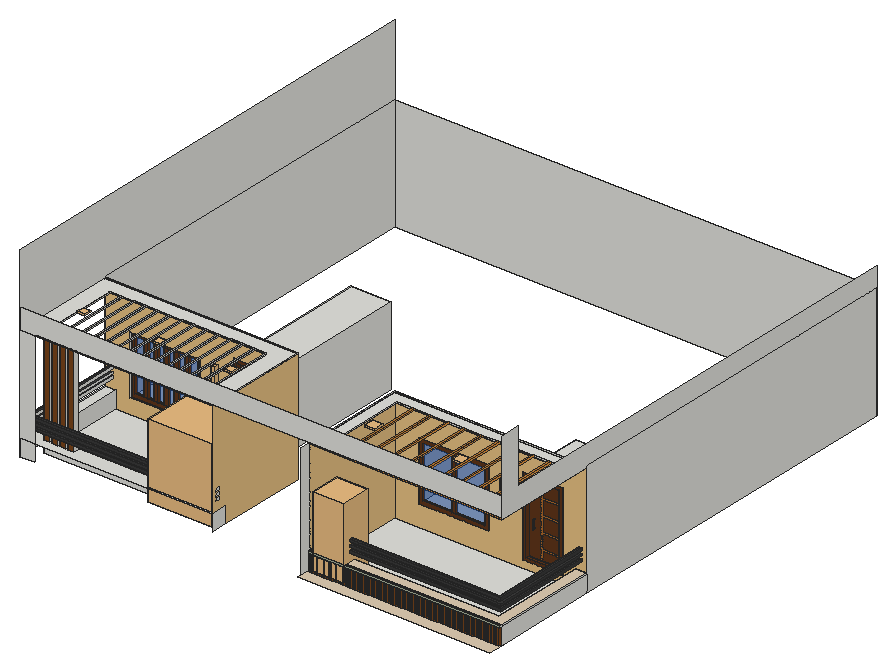
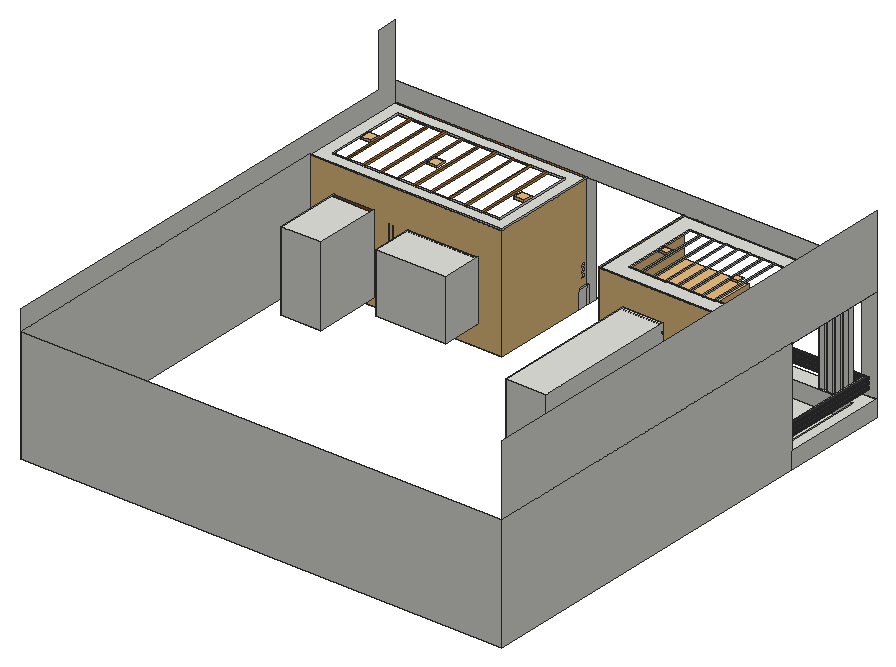
# SketchUp Ruby script. Lengths in inches.
U = 1.inch
M = Sketchup.active_model
def pt(a) = Geom::Point3d.new(a.map { |v| v * U })
def face(e, loops, mat)
  f = e.add_face(loops[0].map { |a| pt(a) })
  loops[1..].each { |l| e.add_face(l.map { |a| pt(a) }).erase! }
  f.material = f.back_material = mat if mat
  f
end
# faces: each face lists its corners as indices into pts; further lists are holes
def faces(e, pts, list, mat = nil) = list.each { |f| face(e, (f[0].is_a?(Array) ? f : [f]).map { |l| l.map { |i| pts[i] } }, mat) }
# xy, xz, yz: faces in a plane at the given z, y or x. An outline is a flat list of corners, or four numbers for a rectangle; further outlines are holes
def ring(l) = l.size == 4 ? [[l[0], l[1]], [l[2], l[1]], [l[2], l[3]], [l[0], l[3]]] : l.each_slice(2).to_a
def flat(e, list, mat, &to3) = list.each { |f| face(e, (f[0].is_a?(Array) ? f : [f]).map { |l| ring(l).map { |u, v| to3.(u, v) } }, mat) }
def xy(e, z, list, mat = nil) = flat(e, list, mat) { |x, y| [x, y, z] }
def xz(e, y, list, mat = nil) = flat(e, list, mat) { |x, z| [x, y, z] }
def yz(e, x, list, mat = nil) = flat(e, list, mat) { |y, z| [x, y, z] }
def lines(e, pts, list) = list.each { |a, b| e.add_line(pt(pts[a]), pt(pts[b])) }
# prism: a flat outline (further loops are holes) pulled along v
def prism(e, loops, v, mat = nil)
  f = face(e, loops, mat); d = Geom::Vector3d.new(v.map { |x| x * U })
  f.pushpull(f.normal.samedirection?(d) ? d.length : -d.length)
end
def box(e, o, s, mat = nil) = prism(e, [[o, [o[0] + s[0], o[1], o[2]], [o[0] + s[0], o[1] + s[1], o[2]], [o[0], o[1] + s[1], o[2]]]], [0, 0, s[2]], mat)
def at(x, y, z, deg = 0) = Geom::Transformation.translation(pt([x, y, z])) * Geom::Transformation.rotation(ORIGIN, Z_AXIS, deg.degrees)
def axes(o, x, y, z) = Geom::Transformation.new([*x, 0, *y, 0, *z, 0, *pt(o).to_a, 1])
def part(name) = M.definitions.add(name)
# library, detail: a bought-in or finely detailed component or shape, given as its bounding box
def library(name, o, s) = part(name).tap { |d| box(d.entities, o, s) }
def detail(e, o, s) = box(e.add_group.entities, o, s)
def put(e, d, t, mat = nil) = e.add_instance(d, t).tap { |i| i.material = mat if mat }
def group(e, t, mat = nil) = e.add_group.tap { |g| g.transformation = t; g.material = mat if mat }.entities
root = M.entities
M.materials.add("Generic\#1").color = [121, 68, 27]
M.materials.add("Generic\#4").color = [232, 149, 60]
M.materials.add("Generic\#5").color = [233, 194, 132]
M.materials.add("Generic\#6").color = [223, 205, 179]
M.materials.add("Generic\#8").color = [168, 180, 155]
M.materials.add("[Color M05]").color = [114, 114, 114]
M.materials.add("[Color M07]").color = [58, 58, 58]
M.materials.add("[Translucent Glass Blue]").color = [28, 83, 181]
M.materials["[Translucent Glass Blue]"].alpha = 0.5
M.materials.add("[Wood Bamboo]").color = [177, 105, 43]
M.materials.add("[Wood Cherry Original]").color = [96, 54, 26]
c1 = part("Group\#10")
xy(c1.entities,17.5625,[[0,0,2,2]])
xz(c1.entities,0,[[0,0,2,17.5625]])
yz(c1.entities,2,[[0,0,2,17.5625]])
c2 = library("Group_2",[-1.28,-0.39,0],[21.22,20.51,48.44])
c3 = library("Flora+17",[-57.52,158.6,-38.64],[66.99,62.88,77.28])
c4 = part("Group\#5")
xy(c4.entities,0,[[0,0,41.8125,3.4375]],"[Wood Cherry Original]")
xy(c4.entities,3.53,[[3.53,0,38.28,3.4375]],"[Wood Cherry Original]")
xy(c4.entities,31.39,[[9.28,1.32,9.97,3.4375]])
xy(c4.entities,32.05,[[9.29,1.98,9.98,3.4375]],"[Color M05]")
xy(c4.entities,39.77,[[9.29,1.98,9.98,3.4375]])
xy(c4.entities,40.43,[[9.28,1.32,9.97,3.4375]],"[Color M05]")
xy(c4.entities,79.47,[[3.53,0,38.28,3.4375]],"[Wood Cherry Original]")
xy(c4.entities,83,[[0,0,41.8125,3.4375]],"[Wood Cherry Original]")
xz(c4.entities,0,[[[0,0,41.8125,83],[3.53,3.53,38.28,79.47]]],"[Wood Cherry Original]")
xz(c4.entities,1.32,[[9.28,31.39,9.97,40.43]],"[Color M05]")
xz(c4.entities,1.98,[[9.29,32.05,9.98,39.77]],"[Color M05]")
xz(c4.entities,3.4375,[[9.29,39.77,9.28,40.43,9.97,40.43,9.98,39.77]])
xz(c4.entities,3.4375,[[16.22,3.53,17.74,3.53,17.74,13.29,38.28,13.29,38.28,15.09,17.74,15.09,17.74,29.41,38.28,29.41,38.28,31.22,17.74,31.22,17.74,45.54,38.28,45.54,38.28,47.34,17.74,47.34,17.74,61.66,38.28,61.66,38.28,63.47,17.74,63.47,17.74,79.47,16.22,79.47]],"[Wood Bamboo]")
xz(c4.entities,3.4375,[[[0,0,41.8125,83],[3.53,3.53,38.28,79.47]],[[3.53,3.53,16.22,79.47],[9.29,39.77,9.28,40.43,9.97,40.43,9.98,39.77],[9.28,31.39,9.29,32.05,9.98,32.05,9.97,31.39]],[17.74,3.53,38.28,13.29],[17.74,15.09,38.28,29.41],[17.74,31.22,38.28,45.54],
  [17.74,47.34,38.28,61.66],[17.74,63.47,38.28,79.47]],"[Wood Cherry Original]")
yz(c4.entities,0,[[0,0,3.4375,83]],"[Wood Cherry Original]")
yz(c4.entities,3.53,[[0,3.53,3.4375,79.47]],"[Wood Cherry Original]")
yz(c4.entities,38.28,[[0,3.53,3.4375,79.47]],"[Wood Cherry Original]")
yz(c4.entities,41.8125,[[0,0,3.4375,83]],"[Wood Cherry Original]")
p = [[9.28,1.32,40.43],[9.29,1.98,39.77],[9.29,1.98,32.05],[9.28,1.32,31.39],[9.29,3.4375,32.05],[9.28,3.4375,31.39],
  [9.98,1.98,39.77],[9.97,1.32,40.43],[9.97,1.32,31.39],[9.98,1.98,32.05],[9.97,3.4375,31.39],[9.98,3.4375,32.05],
  [9.28,3.4375,40.43],[9.29,3.4375,39.77],[9.98,3.4375,39.77],[9.97,3.4375,40.43],[9.625,3.4375,40.13],[9.625,1.625,40.13],
  [9.625,1.625,31.69],[9.625,3.4375,31.69]]
faces(c4.entities,p,[[0,1,2,3],[3,2,4,5],[6,7,8,9],[9,8,10,11],[12,13,1,0],[14,15,7,6]],"[Color M05]")
lines(c4.entities,p,[[16,17],[18,19],[17,18]])
c5 = part("Group\#3")
xy(c5.entities,0,[[0,0,81.86,2.5]],"[Wood Cherry Original]")
xy(c5.entities,4.12,[[4.12,0,13.68,2.5],[13.68,0,18.93,2.5],[18.93,0,25.68,2.5],[25.68,0,30.93,2.5],[30.93,0,37.68,2.5],
  [37.68,0,42.93,2.5],[42.93,0,49.68,2.5],[49.68,0,54.93,2.5],[54.93,0,61.68,2.5],[61.68,0,66.93,2.5],
  [66.93,0,77.74,2.5]],"[Wood Cherry Original]")
xy(c5.entities,66.49,[[4.12,0,13.68,2.5],[13.68,0,18.93,2.5],[18.93,0,25.68,2.5],[25.68,0,30.93,2.5],[30.93,0,37.68,2.5],
  [37.68,0,42.93,2.5],[42.93,0,49.68,2.5],[49.68,0,54.93,2.5],[54.93,0,61.68,2.5],[61.68,0,66.93,2.5],
  [66.93,0,77.74,2.5]],"[Wood Cherry Original]")
xy(c5.entities,70.61,[[0,0,81.86,2.5]],"[Wood Cherry Original]")
xz(c5.entities,0,[[[0,0,81.86,70.61],[4.12,4.12,77.74,66.49]],[13.68,4.12,18.93,66.49],[25.68,4.12,30.93,66.49],[37.68,4.12,42.93,66.49],[49.68,4.12,54.93,66.49],
  [61.68,4.12,66.93,66.49]],"[Wood Cherry Original]")
xz(c5.entities,2.5,[[4.12,4.12,13.68,66.49],[18.93,4.12,25.68,66.49],[30.93,4.12,37.68,66.49],[42.93,4.12,49.68,66.49],[54.93,4.12,61.68,66.49],
  [66.93,4.12,77.74,66.49]],"[Translucent Glass Blue]")
xz(c5.entities,2.5,[[[0,0,81.86,70.61],[4.12,4.12,77.74,66.49]]],"[Wood Cherry Original]")
yz(c5.entities,0,[[0,0,2.5,70.61]],"[Wood Cherry Original]")
yz(c5.entities,4.12,[[0,4.12,2.5,66.49]],"[Wood Cherry Original]")
yz(c5.entities,13.68,[[0,4.12,2.5,66.49]],"[Wood Cherry Original]")
yz(c5.entities,18.93,[[0,4.12,2.5,66.49]],"[Wood Cherry Original]")
yz(c5.entities,25.68,[[0,4.12,2.5,66.49]],"[Wood Cherry Original]")
yz(c5.entities,30.93,[[0,4.12,2.5,66.49]],"[Wood Cherry Original]")
yz(c5.entities,37.68,[[0,4.12,2.5,66.49]],"[Wood Cherry Original]")
yz(c5.entities,42.93,[[0,4.12,2.5,66.49]],"[Wood Cherry Original]")
yz(c5.entities,49.68,[[0,4.12,2.5,66.49]],"[Wood Cherry Original]")
yz(c5.entities,54.93,[[0,4.12,2.5,66.49]],"[Wood Cherry Original]")
yz(c5.entities,61.68,[[0,4.12,2.5,66.49]],"[Wood Cherry Original]")
yz(c5.entities,66.93,[[0,4.12,2.5,66.49]],"[Wood Cherry Original]")
yz(c5.entities,77.74,[[0,4.12,2.5,66.49]],"[Wood Cherry Original]")
yz(c5.entities,81.86,[[0,0,2.5,70.61]],"[Wood Cherry Original]")
c6 = part("Group\#4")
xy(c6.entities,0,[[0,0,73.625,2.0625]],"[Wood Cherry Original]")
xy(c6.entities,3.98,[[35.0625,0,38.75,2.0625]])
xy(c6.entities,3.98,[[3.98,0,35.0625,2.0625],[38.75,0,69.64,2.0625]],"[Wood Cherry Original]")
xy(c6.entities,58.39,[[35.0625,0,38.75,2.0625]])
xy(c6.entities,58.39,[[3.98,0,35.0625,2.0625],[38.75,0,69.64,2.0625]],"[Wood Cherry Original]")
xy(c6.entities,62.375,[[0,0,73.625,2.0625]],"[Wood Cherry Original]")
xz(c6.entities,0,[[[0,0,73.625,62.375],[3.98,3.98,69.64,58.39]],[35.0625,3.98,38.75,58.39]],"[Wood Cherry Original]")
xz(c6.entities,2.0625,[[[0,0,73.625,62.375],[3.98,3.98,69.64,58.39]]])
xz(c6.entities,2.0625,[[3.98,3.98,35.0625,58.39],[38.75,3.98,69.64,58.39]],"[Translucent Glass Blue]")
yz(c6.entities,0,[[0,0,2.0625,62.375]],"[Wood Cherry Original]")
yz(c6.entities,3.98,[[0,3.98,2.0625,58.39]],"[Wood Cherry Original]")
yz(c6.entities,35.0625,[[0,3.98,2.0625,58.39]],"[Wood Cherry Original]")
yz(c6.entities,38.75,[[0,3.98,2.0625,58.39]],"[Wood Cherry Original]")
yz(c6.entities,69.64,[[0,3.98,2.0625,58.39]],"[Wood Cherry Original]")
yz(c6.entities,73.625,[[0,0,2.0625,62.375]],"[Wood Cherry Original]")
c7 = library("Lamp Wall Outdoor 94-02",[-1.89,-4.65,-3.17],[3.78,4.65,6.35])
c8 = library("Tlon Light 450 Ceiling 152 006",[-8.86,-8.86,-3.78],[17.72,17.72,3.56])
xy(root,422.625,[[306.09,52.5625,308.09,54.5625],[306.09,54.5625,306.09,65.5625,496.1875,65.5625,496.1875,166.1875,507.875,166.1875,507.875,54.5625],[306.09,65.5625,496.1875,166.1875],[13.4375,71.3125,204.09,166.1875]])
xy(root,422.625,[[306.09,39.375,507.875,39.375,507.875,54.5625,308.09,54.5625,308.09,52.5625,306.09,52.5625]],"Generic\#6")
xy(root,430.43,[[440.99,166.1875,482.8,235.75]])
xy(root,430.93,[[137.36,166.1875,179.17,320.375]])
xy(root,438.15,[[27.78,166.1875,101.4,224.375]])
xy(root,440.1875,[[306.09,51.8125,308.09,54.5625],[308.09,51.8125,507.875,54.5625],[[2.3125,54.5625,204.09,54.5625,204.09,71.3125,13.4375,71.3125,13.4375,166.1875,2.3125,166.1875],[19.41,64.07,25.6,69.2],[27.85,64.07,34.03,69.2],[36.28,64.07,42.47,69.2],[44.72,64.07,50.91,69.2]],[306.09,54.5625,306.09,65.5625,496.1875,65.5625,496.1875,166.1875,507.875,166.1875,507.875,54.5625]])
xy(root,441.875,[[306.09,54.5625,507.875,54.5625,507.875,166.1875,496.1875,166.1875,496.1875,65.5625,306.09,65.5625]],"Generic\#6")
xy(root,441.875,[[306.09,51.8125,507.875,54.5625]],"Generic\#8")
xy(root,444.9,[[331.4,166.1875,405.03,208.8125]])
xy(root,449.75,[[6.99,59.18,6.99,166.1875,10.24,166.1875,10.24,62.43,204.09,62.43,204.09,59.18]],"[Color M07]")
xy(root,450.64,[[306.09,58.77,306.09,61.77,500.32,61.77,500.32,166.1875,503.32,166.1875,503.32,58.77]],"[Color M07]")
xy(root,452.5,[[6.99,59.18,204.09,59.18,204.09,62.43,10.24,62.43,10.24,166.1875,6.99,166.1875]],"[Color M07]")
xy(root,453.2,[[306.09,58.77,503.32,58.77,503.32,166.1875,500.32,166.1875,500.32,61.77,306.09,61.77]],"[Color M07]")
xy(root,454,[[6.99,59.18,6.99,166.1875,10.24,166.1875,10.24,62.43,204.09,62.43,204.09,59.18]],"[Color M07]")
xy(root,456.01,[[306.09,58.77,306.09,61.77,500.32,61.77,500.32,166.1875,503.32,166.1875,503.32,58.77]],"[Color M07]")
xy(root,456.75,[[6.99,59.18,204.09,59.18,204.09,62.43,10.24,62.43,10.24,166.1875,6.99,166.1875]],"[Color M07]")
xy(root,458.58,[[306.09,58.77,503.32,58.77,503.32,166.1875,500.32,166.1875,500.32,61.77,306.09,61.77]],"[Color M07]")
xy(root,458.75,[[6.99,59.18,6.99,166.1875,10.24,166.1875,10.24,62.43,204.09,62.43,204.09,59.18]],"[Color M07]")
xy(root,461.2,[[306.09,58.77,306.09,61.77,500.32,61.77,500.32,166.1875,503.32,166.1875,503.32,58.77]],"[Color M07]")
xy(root,461.5,[[6.99,59.18,204.09,59.18,204.09,62.43,10.24,62.43,10.24,166.1875,6.99,166.1875]],"[Color M07]")
xy(root,463.76,[[306.09,58.77,503.32,58.77,503.32,166.1875,500.32,166.1875,500.32,61.77,306.09,61.77]],"[Color M07]")
xy(root,500.53,[[27.78,166.1875,101.4,224.375]])
xy(root,507.28,[[331.4,166.1875,405.03,208.8125]])
xy(root,513.43,[[440.99,166.1875,482.8,235.75]])
xy(root,513.93,[[137.36,166.1875,179.17,320.375]])
xy(root,541,[[19.41,64.07,25.6,69.2],[27.85,64.07,34.03,69.2],[36.28,64.07,42.47,69.2],[44.72,64.07,50.91,69.2]])
xy(root,541.1875,[[[306.09,54.5625,507.875,166.1875],[319.4375,67.9,494.53,152.84]]])
xy(root,541.1875,[[336.375,67.9,338.375,152.84],[354.1875,67.9,356.1875,152.84],[372,67.9,374,152.84],[389.8125,67.9,391.8125,152.84],[407.625,67.9,409.625,152.84],
  [425.4375,67.9,427.4375,152.84],[443.25,67.9,445.25,152.84],[461.0625,67.9,463.0625,152.84],[478.875,67.9,480.875,152.84]],"Generic\#4")
xy(root,541.6875,[[[2.3125,54.5625,204.09,166.1875],[18.65,70.9,186.4,149.85]],[18.65,70.9,20.65,149.85],[31.4,70.9,33.4,149.85],[44.15,70.9,46.15,149.85],[56.9,70.9,58.9,149.85],
  [69.65,70.9,71.65,149.85],[82.4,70.9,84.4,149.85],[95.15,70.9,97.15,149.85],[107.9,70.9,109.9,149.85],[120.65,70.9,122.65,149.85],
  [133.4,70.9,135.4,149.85],[146.15,70.9,148.15,149.85],[158.9,70.9,160.9,149.85],[171.65,70.9,173.65,149.85],[184.4,70.9,186.4,149.85]])
xz(root,51.8125,[[306.09,440.1875,507.875,441.875]],"Generic\#8")
xz(root,54.5625,[[2.3125,422.625,17.125,440.1875],[306.09,422.625,308.09,440.1875],[308.09,422.625,507.875,440.1875],[2.3125,440.1875,17.125,541.6875],[306.09,440.1875,507.875,441.875],
  [2.3125,541.6875,2.3125,563.5,507.875,563.5,507.875,542.625,17.125,542.625,17.125,541.6875],[17.125,541.6875,204.09,542.625]])
xz(root,54.5625,[[306.09,541.1875,507.875,542.625]],"Generic\#4")
xz(root,58.77,[[306.09,450.64,503.32,453.2],[306.09,456.01,503.32,458.58],[306.09,461.2,503.32,463.76]],"[Color M07]")
xz(root,59.18,[[6.99,449.75,204.09,452.5],[6.99,454,204.09,456.75],[6.99,458.75,204.09,461.5]],"[Color M07]")
xz(root,61.77,[[306.09,450.64,500.32,453.2],[306.09,456.01,500.32,458.58],[306.09,461.2,500.32,463.76]],"[Color M07]")
xz(root,62.43,[[10.24,449.75,204.09,452.5],[10.24,454,204.09,456.75],[10.24,458.75,204.09,461.5]],"[Color M07]")
xz(root,64.07,[[19.41,440.1875,25.6,541],[27.85,440.1875,34.03,541],[36.28,440.1875,42.47,541],[44.72,440.1875,50.91,541]],"Generic\#1")
xz(root,65.5625,[[306.09,422.625,496.1875,440.1875],[306.09,440.1875,496.1875,441.875]])
xz(root,67.9,[[319.4375,541.1875,336.375,542.625],[338.375,541.1875,354.1875,542.625],[356.1875,541.1875,372,542.625],[374,541.1875,389.8125,542.625],[391.8125,541.1875,407.625,542.625],
  [409.625,541.1875,425.4375,542.625],[427.4375,541.1875,443.25,542.625],[445.25,541.1875,461.0625,542.625],[463.0625,541.1875,478.875,542.625],[480.875,541.1875,494.53,542.625]])
xz(root,69.2,[[19.41,440.1875,25.6,541],[27.85,440.1875,34.03,541],[36.28,440.1875,42.47,541],[44.72,440.1875,50.91,541]])
xz(root,70.9,[[20.65,541.6875,31.4,542.625],[33.4,541.6875,44.15,542.625],[46.15,541.6875,56.9,542.625],[58.9,541.6875,69.65,542.625],[71.65,541.6875,82.4,542.625],
  [84.4,541.6875,95.15,542.625],[97.15,541.6875,107.9,542.625],[109.9,541.6875,120.65,542.625],[122.65,541.6875,133.4,542.625],[135.4,541.6875,146.15,542.625],
  [148.15,541.6875,158.9,542.625],[160.9,541.6875,171.65,542.625],[173.65,541.6875,184.4,542.625]])
xz(root,71.3125,[[13.4375,422.625,204.09,440.1875]])
xz(root,149.85,[[20.65,541.6875,31.4,542.625],[33.4,541.6875,44.15,542.625],[46.15,541.6875,56.9,542.625],[58.9,541.6875,69.65,542.625],[71.65,541.6875,82.4,542.625],
  [84.4,541.6875,95.15,542.625],[97.15,541.6875,107.9,542.625],[109.9,541.6875,120.65,542.625],[122.65,541.6875,133.4,542.625],[135.4,541.6875,146.15,542.625],
  [148.15,541.6875,158.9,542.625],[160.9,541.6875,171.65,542.625],[173.65,541.6875,184.4,542.625]])
xz(root,152.84,[[319.4375,541.1875,336.375,542.625],[338.375,541.1875,354.1875,542.625],[356.1875,541.1875,372,542.625],[374,541.1875,389.8125,542.625],[391.8125,541.1875,407.625,542.625],
  [409.625,541.1875,425.4375,542.625],[427.4375,541.1875,443.25,542.625],[445.25,541.1875,461.0625,542.625],[463.0625,541.1875,478.875,542.625],[480.875,541.1875,494.53,542.625]])
xz(root,166.1875,[[496.1875,440.1875,507.875,441.875],[306.09,541.1875,507.875,542.625],[2.3125,541.6875,204.09,542.625]])
xz(root,166.1875,[[[13.4375,422.625,204.09,422.625,204.09,541.6875,2.3125,541.6875,2.3125,440.1875,13.4375,440.1875],[27.78,438.15,101.4,500.53],[137.36,430.93,179.17,513.93],[6.99,458.75,10.24,461.5],[6.99,454,10.24,456.75],[6.99,449.75,10.24,452.5]],[[306.09,422.625,496.1875,422.625,496.1875,441.875,507.875,441.875,507.875,541.1875,306.09,541.1875],[331.4,444.9,405.03,507.28],[440.99,430.43,482.8,513.43],[500.32,450.64,503.32,453.2],[500.32,456.01,503.32,458.58],[500.32,461.2,503.32,463.76]]],"Generic\#5")
xz(root,208.8125,[[331.4,444.9,405.03,507.28]])
xz(root,224.375,[[27.78,438.15,101.4,500.53]])
xz(root,235.75,[[440.99,430.43,482.8,513.43]])
xz(root,320.375,[[137.36,430.93,179.17,513.93]])
xz(root,546.8125,[[2.3125,422.625,507.875,542.625]])
yz(root,2.3125,[[54.5625,422.625,166.1875,440.1875],[166.1875,422.625,546.8125,542.625],[54.5625,541.6875,54.5625,617.375,546.8125,617.375,546.8125,542.625,166.1875,542.625,166.1875,541.6875]])
yz(root,6.99,[[59.18,449.75,166.1875,452.5],[59.18,454,166.1875,456.75],[59.18,458.75,166.1875,461.5]],"[Color M07]")
yz(root,10.24,[[62.43,449.75,166.1875,452.5],[62.43,454,166.1875,456.75],[62.43,458.75,166.1875,461.5]])
yz(root,13.4375,[[71.3125,422.625,166.1875,440.1875]])
yz(root,19.41,[[64.07,440.1875,69.2,541]])
yz(root,20.65,[[70.9,541.6875,149.85,542.625]])
yz(root,25.6,[[64.07,440.1875,69.2,541]])
yz(root,27.78,[[166.1875,438.15,224.375,500.53]])
yz(root,27.85,[[64.07,440.1875,69.2,541]])
yz(root,31.4,[[70.9,541.6875,149.85,542.625]])
yz(root,33.4,[[70.9,541.6875,149.85,542.625]])
yz(root,34.03,[[64.07,440.1875,69.2,541]])
yz(root,36.28,[[64.07,440.1875,69.2,541]])
yz(root,42.47,[[64.07,440.1875,69.2,541]])
yz(root,44.15,[[70.9,541.6875,149.85,542.625]])
yz(root,44.72,[[64.07,440.1875,69.2,541]])
yz(root,46.15,[[70.9,541.6875,149.85,542.625]])
yz(root,50.91,[[64.07,440.1875,69.2,541]])
yz(root,56.9,[[70.9,541.6875,149.85,542.625]])
yz(root,58.9,[[70.9,541.6875,149.85,542.625]])
yz(root,69.65,[[70.9,541.6875,149.85,542.625]])
yz(root,71.65,[[70.9,541.6875,149.85,542.625]])
yz(root,82.4,[[70.9,541.6875,149.85,542.625]])
yz(root,84.4,[[70.9,541.6875,149.85,542.625]])
yz(root,95.15,[[70.9,541.6875,149.85,542.625]])
yz(root,97.15,[[70.9,541.6875,149.85,542.625]])
yz(root,101.4,[[166.1875,438.15,224.375,500.53]])
yz(root,107.9,[[70.9,541.6875,149.85,542.625]])
yz(root,109.9,[[70.9,541.6875,149.85,542.625]])
yz(root,120.65,[[70.9,541.6875,149.85,542.625]])
yz(root,122.65,[[70.9,541.6875,149.85,542.625]])
yz(root,133.4,[[70.9,541.6875,149.85,542.625]])
yz(root,135.4,[[70.9,541.6875,149.85,542.625]])
yz(root,137.36,[[166.1875,430.93,320.375,513.93]])
yz(root,146.15,[[70.9,541.6875,149.85,542.625]])
yz(root,148.15,[[70.9,541.6875,149.85,542.625]])
yz(root,158.9,[[70.9,541.6875,149.85,542.625]])
yz(root,160.9,[[70.9,541.6875,149.85,542.625]])
yz(root,171.65,[[70.9,541.6875,149.85,542.625]])
yz(root,173.65,[[70.9,541.6875,149.85,542.625]])
yz(root,179.17,[[166.1875,430.93,320.375,513.93]])
yz(root,184.4,[[70.9,541.6875,149.85,542.625]])
yz(root,204.09,[[54.5625,422.625,71.3125,440.1875],[59.18,449.75,62.43,452.5],[59.18,454,62.43,456.75],[59.18,458.75,62.43,461.5],[54.5625,541.6875,166.1875,542.625]])
yz(root,204.09,[[[71.3125,422.625,71.3125,440.1875,54.5625,440.1875,54.5625,541.6875,166.1875,541.6875,166.1875,422.625],[59.18,458.75,62.43,461.5],[59.18,454,62.43,456.75],[59.18,449.75,62.43,452.5]]],"Generic\#5")
yz(root,306.09,[[43.625,422.625,52.5625,422.625,52.5625,440.1875,51.8125,440.1875,51.8125,441.875,54.5625,441.875,54.5625,542.625,43.625,542.625],[52.5625,422.625,54.5625,440.1875],[54.5625,422.625,65.5625,440.1875],[51.8125,440.1875,54.5625,441.875],[54.5625,440.1875,65.5625,441.875],
  [58.77,450.64,61.77,453.2],[58.77,456.01,61.77,458.58],[58.77,461.2,61.77,463.76],[54.5625,541.1875,166.1875,542.625]])
yz(root,306.09,[[[65.5625,422.625,166.1875,422.625,166.1875,541.1875,54.5625,541.1875,54.5625,441.875,65.5625,441.875],[58.77,461.2,61.77,463.76],[58.77,456.01,61.77,458.58],[58.77,450.64,61.77,453.2]]],"Generic\#5")
yz(root,319.4375,[[67.9,541.1875,152.84,542.625]])
yz(root,331.4,[[166.1875,444.9,208.8125,507.28]])
yz(root,336.375,[[67.9,541.1875,152.84,542.625]],"Generic\#4")
yz(root,338.375,[[67.9,541.1875,152.84,542.625]],"Generic\#4")
yz(root,354.1875,[[67.9,541.1875,152.84,542.625]],"Generic\#4")
yz(root,356.1875,[[67.9,541.1875,152.84,542.625]],"Generic\#4")
yz(root,372,[[67.9,541.1875,152.84,542.625]],"Generic\#4")
yz(root,374,[[67.9,541.1875,152.84,542.625]],"Generic\#4")
yz(root,389.8125,[[67.9,541.1875,152.84,542.625]],"Generic\#4")
yz(root,391.8125,[[67.9,541.1875,152.84,542.625]],"Generic\#4")
yz(root,405.03,[[166.1875,444.9,208.8125,507.28]])
yz(root,407.625,[[67.9,541.1875,152.84,542.625]],"Generic\#4")
yz(root,409.625,[[67.9,541.1875,152.84,542.625]],"Generic\#4")
yz(root,425.4375,[[67.9,541.1875,152.84,542.625]],"Generic\#4")
yz(root,427.4375,[[67.9,541.1875,152.84,542.625]],"Generic\#4")
yz(root,440.99,[[166.1875,430.43,235.75,513.43]])
yz(root,443.25,[[67.9,541.1875,152.84,542.625]],"Generic\#4")
yz(root,445.25,[[67.9,541.1875,152.84,542.625]],"Generic\#4")
yz(root,461.0625,[[67.9,541.1875,152.84,542.625]],"Generic\#4")
yz(root,463.0625,[[67.9,541.1875,152.84,542.625]],"Generic\#4")
yz(root,478.875,[[67.9,541.1875,152.84,542.625]],"Generic\#4")
yz(root,480.875,[[67.9,541.1875,152.84,542.625]],"Generic\#4")
yz(root,482.8,[[166.1875,430.43,235.75,513.43]])
yz(root,494.53,[[67.9,541.1875,152.84,542.625]])
yz(root,496.1875,[[65.5625,422.625,166.1875,440.1875],[65.5625,440.1875,166.1875,441.875]])
yz(root,500.32,[[61.77,450.64,166.1875,453.2],[61.77,456.01,166.1875,458.58],[61.77,461.2,166.1875,463.76]],"[Color M07]")
yz(root,503.32,[[58.77,450.64,166.1875,453.2],[58.77,456.01,166.1875,458.58],[58.77,461.2,166.1875,463.76]],"[Color M07]")
yz(root,507.875,[[54.5625,422.625,166.1875,440.1875],[166.1875,422.625,546.8125,542.625],[51.8125,440.1875,54.5625,441.875],[54.5625,440.1875,166.1875,441.875],[54.5625,541.1875,166.1875,541.1875,166.1875,542.625,546.8125,542.625,546.8125,563.5,76.4375,563.5,76.4375,619.375,54.5625,619.375]])
p = [[2.3125,166.1875,422.625],[13.4375,166.1875,422.625],[306.09,60.0625,451.9375],[502.03,60.0625,451.9375],[502.03,166.1875,451.9375],[306.09,60.0625,457.25],
  [502.03,60.0625,457.25],[502.03,166.1875,457.25],[306.09,60.0625,462.5625],[502.03,60.0625,462.5625],[502.03,166.1875,462.5625],[7.875,166.1875,450.9375],
  [7.875,60.0625,450.9375],[204.09,60.0625,450.9375],[7.875,166.1875,460.125],[7.875,60.0625,460.125],[204.09,60.0625,460.125],[7.875,166.1875,455.5],
  [7.875,60.0625,455.5],[204.09,60.0625,455.5]]
lines(root,p,[[0,1],[2,3],[4,3],[5,6],[7,6],[8,9],[10,9],[11,12],[13,12],[14,15],[16,15],[17,18],
  [19,18]])
put(root,c1,at(306.09,52.5625,422.625),"Generic\#1")
put(root,c1,at(308.59,52.5625,422.625),"Generic\#1")
put(root,c1,at(311.09,52.5625,422.625),"Generic\#1")
put(root,c1,at(313.59,52.5625,422.625),"Generic\#1")
put(root,c1,at(316.09,52.5625,422.625),"Generic\#1")
put(root,c1,at(318.59,52.5625,422.625),"Generic\#1")
put(root,c1,at(321.09,52.5625,422.625),"Generic\#1")
put(root,c1,at(323.59,52.5625,422.625),"Generic\#1")
put(root,c1,at(326.09,52.5625,422.625),"Generic\#1")
put(root,c1,at(328.59,52.5625,422.625),"Generic\#1")
put(root,c1,at(331.09,52.5625,422.625),"Generic\#1")
put(root,c1,at(333.59,52.5625,422.625),"Generic\#1")
put(root,c1,at(336.09,52.5625,422.625),"Generic\#1")
put(root,c1,at(338.59,52.5625,422.625),"Generic\#1")
put(root,c1,at(341.09,52.5625,422.625),"Generic\#1")
put(root,c1,at(343.59,52.5625,422.625),"Generic\#1")
put(root,c1,at(346.09,52.5625,422.625),"Generic\#1")
put(root,c1,at(348.59,52.5625,422.625),"Generic\#1")
put(root,c1,at(351.09,52.5625,422.625),"Generic\#1")
put(root,c1,at(353.59,52.5625,422.625),"Generic\#1")
put(root,c1,at(356.09,52.5625,422.625),"Generic\#1")
put(root,c1,at(358.59,52.5625,422.625),"Generic\#1")
put(root,c1,at(361.09,52.5625,422.625),"Generic\#1")
put(root,c1,at(363.59,52.5625,422.625),"Generic\#1")
put(root,c1,at(366.09,52.5625,422.625),"Generic\#1")
put(root,c1,at(368.59,52.5625,422.625),"Generic\#1")
put(root,c1,at(371.09,52.5625,422.625),"Generic\#1")
put(root,c1,at(373.59,52.5625,422.625),"Generic\#1")
put(root,c1,at(376.09,52.5625,422.625),"Generic\#1")
put(root,c1,at(378.59,52.5625,422.625),"Generic\#1")
put(root,c1,at(381.09,52.5625,422.625),"Generic\#1")
put(root,c1,at(383.59,52.5625,422.625),"Generic\#1")
put(root,c1,at(386.09,52.5625,422.625),"Generic\#1")
put(root,c1,at(388.59,52.5625,422.625),"Generic\#1")
put(root,c1,at(391.09,52.5625,422.625),"Generic\#1")
put(root,c1,at(393.59,52.5625,422.625),"Generic\#1")
put(root,c1,at(396.09,52.5625,422.625),"Generic\#1")
put(root,c1,at(398.59,52.5625,422.625),"Generic\#1")
put(root,c1,at(401.09,52.5625,422.625),"Generic\#1")
put(root,c1,at(403.59,52.5625,422.625),"Generic\#1")
put(root,c1,at(406.09,52.5625,422.625),"Generic\#1")
put(root,c1,at(408.59,52.5625,422.625),"Generic\#1")
put(root,c1,at(411.09,52.5625,422.625),"Generic\#1")
put(root,c1,at(413.59,52.5625,422.625),"Generic\#1")
put(root,c1,at(416.09,52.5625,422.625),"Generic\#1")
put(root,c1,at(418.59,52.5625,422.625),"Generic\#1")
put(root,c1,at(421.09,52.5625,422.625),"Generic\#1")
put(root,c1,at(423.59,52.5625,422.625),"Generic\#1")
put(root,c1,at(426.09,52.5625,422.625),"Generic\#1")
put(root,c1,at(428.59,52.5625,422.625),"Generic\#1")
put(root,c1,at(431.09,52.5625,422.625),"Generic\#1")
put(root,c1,at(433.59,52.5625,422.625),"Generic\#1")
put(root,c1,at(436.09,52.5625,422.625),"Generic\#1")
put(root,c1,at(438.59,52.5625,422.625),"Generic\#1")
put(root,c1,at(441.09,52.5625,422.625),"Generic\#1")
put(root,c1,at(443.59,52.5625,422.625),"Generic\#1")
put(root,c1,at(446.09,52.5625,422.625),"Generic\#1")
put(root,c1,at(448.59,52.5625,422.625),"Generic\#1")
put(root,c1,at(451.09,52.5625,422.625),"Generic\#1")
put(root,c1,at(453.59,52.5625,422.625),"Generic\#1")
put(root,c1,at(456.09,52.5625,422.625),"Generic\#1")
put(root,c1,at(458.59,52.5625,422.625),"Generic\#1")
put(root,c1,at(461.09,52.5625,422.625),"Generic\#1")
put(root,c1,at(463.59,52.5625,422.625),"Generic\#1")
put(root,c1,at(466.09,52.5625,422.625),"Generic\#1")
put(root,c1,at(468.59,52.5625,422.625),"Generic\#1")
put(root,c1,at(471.09,52.5625,422.625),"Generic\#1")
put(root,c1,at(473.59,52.5625,422.625),"Generic\#1")
put(root,c1,at(476.09,52.5625,422.625),"Generic\#1")
put(root,c1,at(478.59,52.5625,422.625),"Generic\#1")
put(root,c1,at(481.09,52.5625,422.625),"Generic\#1")
put(root,c1,at(483.59,52.5625,422.625),"Generic\#1")
put(root,c1,at(486.09,52.5625,422.625),"Generic\#1")
put(root,c1,at(488.59,52.5625,422.625),"Generic\#1")
put(root,c1,at(491.09,52.5625,422.625),"Generic\#1")
put(root,c1,at(493.59,52.5625,422.625),"Generic\#1")
put(root,c1,at(496.09,52.5625,422.625),"Generic\#1")
put(root,c1,at(499.03,52.5625,422.625),"Generic\#1")
put(root,c1,at(501.97,52.5625,422.625),"Generic\#1")
put(root,c1,at(504.91,52.5625,422.625),"Generic\#1")
put(root,c2,axes([313.59,52.5625,424.79],[1.54,0,0],[0,1.54,0],[0,0,1.54]))
put(root,c3,at(192.07,-102.17,464.81))
put(root,c4,at(440.99,166.1875,430.43))
put(root,c4,axes([137.36,166.1875,432.59],[1,0,0],[0,1,0],[0,0,0.98]))
put(root,c5,axes([27.78,168.92,438.15],[0.89936,0,0],[0,0.8633,0],[0,0,0.88057]))
put(root,c6,at(331.4,166.1875,444.9))
put(root,c7,axes([118.9,166.1875,491.3],[1,0,0],[0,1,0],[0,0,3.19]))
put(root,c7,axes([422.9,166.1875,495.67],[1,0,0],[0,1,0],[0,0,3.19]))
put(root,c8,axes([488.21,111.93,542.67],[0.59,0,0],[0,0.59,0],[0,0,0.59]))
put(root,c8,axes([419.46,111.93,542.67],[0.59,0,0],[0,0.59,0],[0,0,0.59]))
put(root,c8,axes([327.65,111.93,542.67],[0.59,0,0],[0,0.59,0],[0,0,0.59]))
put(root,c8,axes([178.9,110.41,543.38],[0.44852,0,0],[0,0.44852,0],[0,0,0.44852]))
put(root,c8,axes([103.78,110.41,543.38],[0.44852,0,0],[0,0.44852,0],[0,0,0.44852]))
put(root,c8,axes([24.625,110.41,543.38],[0.44852,0,0],[0,0.44852,0],[0,0,0.44852]))
